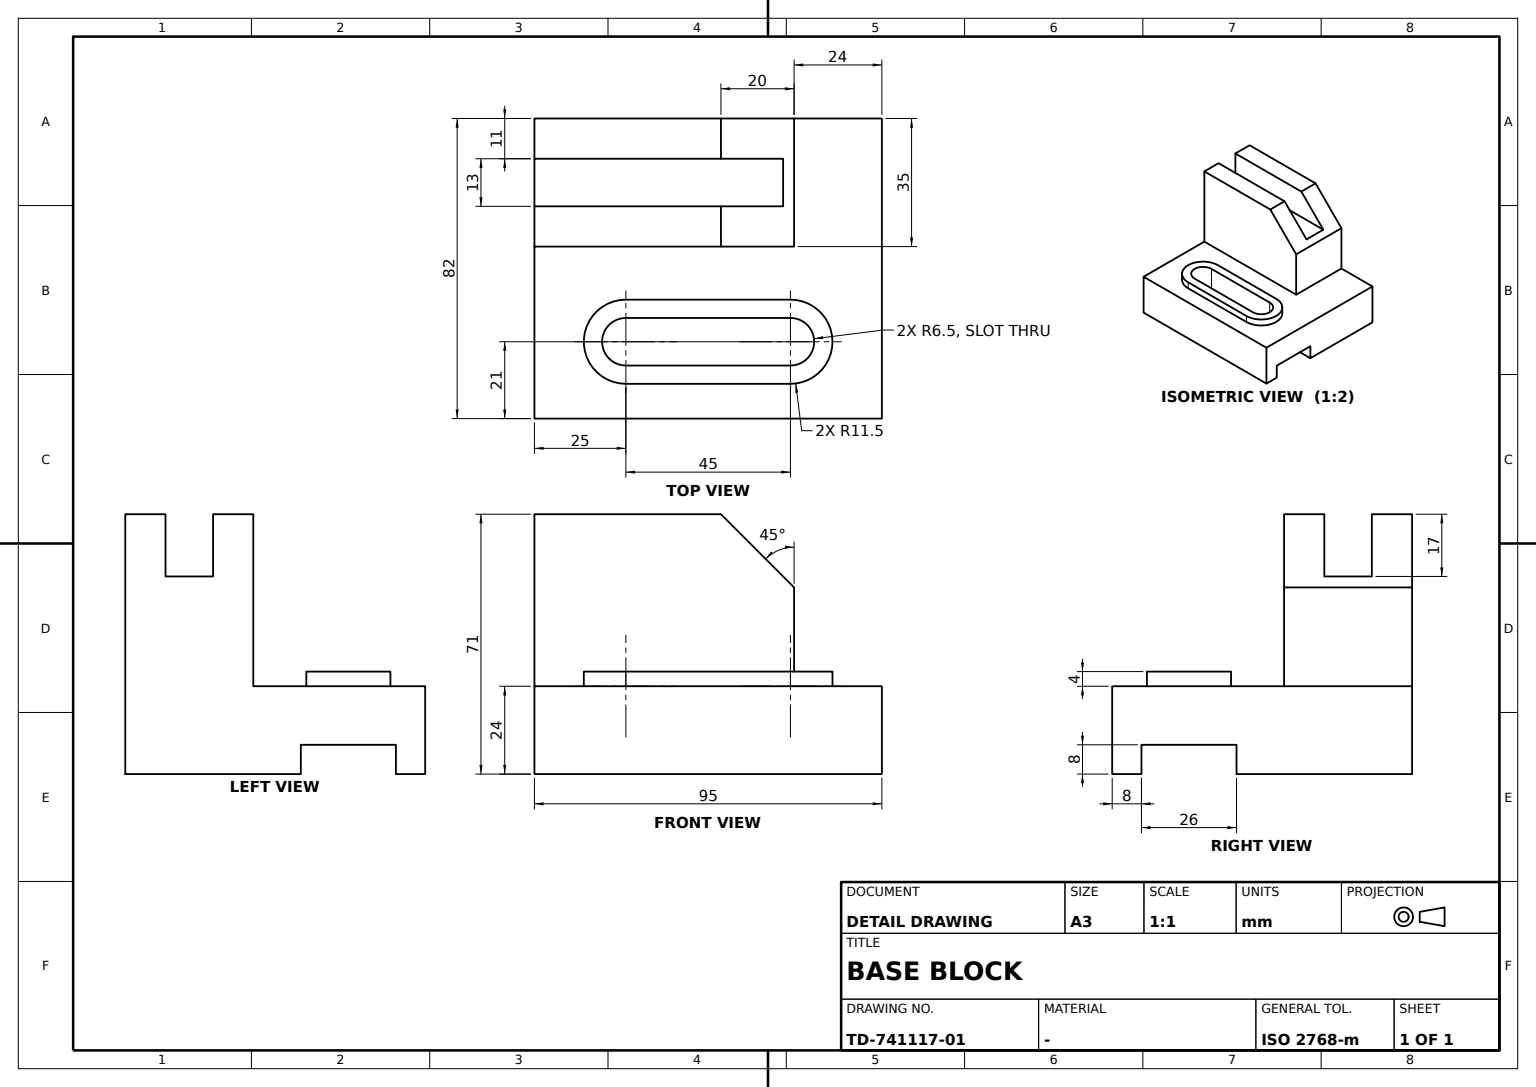
ISO-10303-21;
HEADER;
FILE_DESCRIPTION((''),'2;1');
FILE_NAME('','',(''),(''),'','','');
FILE_SCHEMA(('AUTOMOTIVE_DESIGN'));
ENDSEC;
DATA;
#1=APPLICATION_CONTEXT('');
#2=PRODUCT_CONTEXT('',#1,'mechanical');
#3=PRODUCT('','','',(#2));
#4=PRODUCT_DEFINITION_FORMATION('','',#3);
#5=PRODUCT_DEFINITION_CONTEXT('',#1,'design');
#6=PRODUCT_DEFINITION('','',#4,#5);
#7=PRODUCT_DEFINITION_SHAPE('','',#6);
#8=(LENGTH_UNIT()NAMED_UNIT(*)SI_UNIT(.MILLI.,.METRE.));
#9=(NAMED_UNIT(*)PLANE_ANGLE_UNIT()SI_UNIT($,.RADIAN.));
#10=(NAMED_UNIT(*)SI_UNIT($,.STERADIAN.)SOLID_ANGLE_UNIT());
#11=UNCERTAINTY_MEASURE_WITH_UNIT(LENGTH_MEASURE(0.005),#8,'distance_accuracy_value','');
#12=(GEOMETRIC_REPRESENTATION_CONTEXT(3)GLOBAL_UNCERTAINTY_ASSIGNED_CONTEXT((#11))GLOBAL_UNIT_ASSIGNED_CONTEXT((#8,#9,#10))REPRESENTATION_CONTEXT('',''));
#13=CARTESIAN_POINT('',(95.,34.,8.));
#14=VERTEX_POINT('',#13);
#15=CARTESIAN_POINT('',(0.,34.,8.));
#16=VERTEX_POINT('',#15);
#17=DIRECTION('',(-1.,0.,0.));
#18=VECTOR('',#17,1000.);
#19=LINE('',#15,#18);
#20=EDGE_CURVE('',#14,#16,#19,.T.);
#21=ORIENTED_EDGE('',*,*,#20,.T.);
#22=CARTESIAN_POINT('',(0.,34.,0.));
#23=VERTEX_POINT('',#22);
#24=DIRECTION('',(0.,0.,1.));
#25=VECTOR('',#24,1000.);
#26=LINE('',#22,#25);
#27=EDGE_CURVE('',#23,#16,#26,.T.);
#28=ORIENTED_EDGE('',*,*,#27,.F.);
#29=CARTESIAN_POINT('',(95.,34.,0.));
#30=VERTEX_POINT('',#29);
#31=DIRECTION('',(1.,0.,0.));
#32=VECTOR('',#31,1000.);
#33=LINE('',#22,#32);
#34=EDGE_CURVE('',#23,#30,#33,.T.);
#35=ORIENTED_EDGE('',*,*,#34,.T.);
#36=LINE('',#29,#25);
#37=EDGE_CURVE('',#30,#14,#36,.T.);
#38=ORIENTED_EDGE('',*,*,#37,.T.);
#39=EDGE_LOOP('',(#21,#28,#35,#38));
#40=FACE_BOUND('',#39,.T.);
#41=DIRECTION('',(0.,1.,0.));
#42=AXIS2_PLACEMENT_3D('',#22,#41,#24);
#43=PLANE('',#42);
#44=ADVANCED_FACE('',(#40),#43,.F.);
#45=CARTESIAN_POINT('',(70.,32.5,28.));
#46=VERTEX_POINT('',#45);
#47=CARTESIAN_POINT('',(25.,32.5,28.));
#48=VERTEX_POINT('',#47);
#49=LINE('',#45,#18);
#50=EDGE_CURVE('',#46,#48,#49,.T.);
#51=ORIENTED_EDGE('',*,*,#50,.F.);
#52=CARTESIAN_POINT('',(70.,32.5,24.));
#53=VERTEX_POINT('',#52);
#54=LINE('',#52,#25);
#55=EDGE_CURVE('',#53,#46,#54,.T.);
#56=ORIENTED_EDGE('',*,*,#55,.F.);
#57=CARTESIAN_POINT('',(25.,32.5,24.));
#58=VERTEX_POINT('',#57);
#59=LINE('',#52,#18);
#60=EDGE_CURVE('',#53,#58,#59,.T.);
#61=ORIENTED_EDGE('',*,*,#60,.T.);
#62=LINE('',#57,#25);
#63=EDGE_CURVE('',#58,#48,#62,.T.);
#64=ORIENTED_EDGE('',*,*,#63,.T.);
#65=EDGE_LOOP('',(#51,#56,#61,#64));
#66=FACE_BOUND('',#65,.T.);
#67=AXIS2_PLACEMENT_3D('',#52,#41,#17);
#68=PLANE('',#67);
#69=ADVANCED_FACE('',(#66),#68,.T.);
#70=CARTESIAN_POINT('',(71.,82.,51.));
#71=VERTEX_POINT('',#70);
#72=CARTESIAN_POINT('',(71.,47.,51.));
#73=VERTEX_POINT('',#72);
#74=DIRECTION('',(0.,-1.,0.));
#75=VECTOR('',#74,1000.);
#76=LINE('',#72,#75);
#77=EDGE_CURVE('',#71,#73,#76,.T.);
#78=ORIENTED_EDGE('',*,*,#77,.T.);
#79=CARTESIAN_POINT('',(71.,47.,24.));
#80=VERTEX_POINT('',#79);
#81=LINE('',#79,#25);
#82=EDGE_CURVE('',#80,#73,#81,.T.);
#83=ORIENTED_EDGE('',*,*,#82,.F.);
#84=CARTESIAN_POINT('',(71.,82.,24.));
#85=VERTEX_POINT('',#84);
#86=VECTOR('',#41,1000.);
#87=LINE('',#79,#86);
#88=EDGE_CURVE('',#80,#85,#87,.T.);
#89=ORIENTED_EDGE('',*,*,#88,.T.);
#90=LINE('',#84,#25);
#91=EDGE_CURVE('',#85,#71,#90,.T.);
#92=ORIENTED_EDGE('',*,*,#91,.T.);
#93=EDGE_LOOP('',(#78,#83,#89,#92));
#94=FACE_BOUND('',#93,.T.);
#95=DIRECTION('',(0.,0.,-1.));
#96=AXIS2_PLACEMENT_3D('',#79,#31,#95);
#97=PLANE('',#96);
#98=ADVANCED_FACE('',(#94),#97,.T.);
#99=CARTESIAN_POINT('',(25.,27.5,8.));
#100=VERTEX_POINT('',#99);
#101=CARTESIAN_POINT('',(25.,27.5,28.));
#102=VERTEX_POINT('',#101);
#103=CARTESIAN_POINT('',(25.,27.5,24.));
#104=LINE('',#103,#25);
#105=EDGE_CURVE('',#100,#102,#104,.T.);
#106=ORIENTED_EDGE('',*,*,#105,.T.);
#107=CARTESIAN_POINT('',(25.,14.5,28.));
#108=VERTEX_POINT('',#107);
#109=CARTESIAN_POINT('',(25.,21.,28.));
#110=AXIS2_PLACEMENT_3D('',#109,#95,#41);
#111=CIRCLE('',#110,6.5);
#112=EDGE_CURVE('',#108,#102,#111,.T.);
#113=ORIENTED_EDGE('',*,*,#112,.F.);
#114=CARTESIAN_POINT('',(25.,14.5,8.));
#115=VERTEX_POINT('',#114);
#116=CARTESIAN_POINT('',(25.,14.5,24.));
#117=LINE('',#116,#25);
#118=EDGE_CURVE('',#115,#108,#117,.T.);
#119=ORIENTED_EDGE('',*,*,#118,.F.);
#120=CARTESIAN_POINT('',(25.,21.,8.));
#121=AXIS2_PLACEMENT_3D('',#120,#24,#31);
#122=CIRCLE('',#121,6.5);
#123=EDGE_CURVE('',#100,#115,#122,.T.);
#124=ORIENTED_EDGE('',*,*,#123,.F.);
#125=EDGE_LOOP('',(#106,#113,#119,#124));
#126=FACE_BOUND('',#125,.T.);
#127=CARTESIAN_POINT('',(25.,21.,24.));
#128=AXIS2_PLACEMENT_3D('',#127,#24,#31);
#129=CYLINDRICAL_SURFACE('',#128,6.5);
#130=ADVANCED_FACE('',(#126),#129,.F.);
#131=CARTESIAN_POINT('',(70.,27.5,8.));
#132=VERTEX_POINT('',#131);
#133=CARTESIAN_POINT('',(70.,27.5,28.));
#134=VERTEX_POINT('',#133);
#135=CARTESIAN_POINT('',(70.,27.5,24.));
#136=LINE('',#135,#25);
#137=EDGE_CURVE('',#132,#134,#136,.T.);
#138=ORIENTED_EDGE('',*,*,#137,.F.);
#139=CARTESIAN_POINT('',(76.5,21.,8.));
#140=VERTEX_POINT('',#139);
#141=CARTESIAN_POINT('',(70.,21.,8.));
#142=AXIS2_PLACEMENT_3D('',#141,#24,#31);
#143=CIRCLE('',#142,6.5);
#144=EDGE_CURVE('',#140,#132,#143,.T.);
#145=ORIENTED_EDGE('',*,*,#144,.F.);
#146=CARTESIAN_POINT('',(76.5,21.,28.));
#147=VERTEX_POINT('',#146);
#148=CARTESIAN_POINT('',(76.5,21.,24.));
#149=LINE('',#148,#25);
#150=EDGE_CURVE('',#140,#147,#149,.T.);
#151=ORIENTED_EDGE('',*,*,#150,.T.);
#152=CARTESIAN_POINT('',(70.,21.,28.));
#153=AXIS2_PLACEMENT_3D('',#152,#95,#41);
#154=CIRCLE('',#153,6.5);
#155=EDGE_CURVE('',#134,#147,#154,.T.);
#156=ORIENTED_EDGE('',*,*,#155,.F.);
#157=EDGE_LOOP('',(#138,#145,#151,#156));
#158=FACE_BOUND('',#157,.T.);
#159=CARTESIAN_POINT('',(70.,21.,24.));
#160=AXIS2_PLACEMENT_3D('',#159,#24,#31);
#161=CYLINDRICAL_SURFACE('',#160,6.5);
#162=ADVANCED_FACE('',(#158),#161,.F.);
#163=CARTESIAN_POINT('',(0.,0.,0.));
#164=VERTEX_POINT('',#163);
#165=CARTESIAN_POINT('',(95.,0.,0.));
#166=VERTEX_POINT('',#165);
#167=LINE('',#163,#32);
#168=EDGE_CURVE('',#164,#166,#167,.T.);
#169=ORIENTED_EDGE('',*,*,#168,.T.);
#170=CARTESIAN_POINT('',(95.,0.,24.));
#171=VERTEX_POINT('',#170);
#172=LINE('',#165,#25);
#173=EDGE_CURVE('',#166,#171,#172,.T.);
#174=ORIENTED_EDGE('',*,*,#173,.T.);
#175=CARTESIAN_POINT('',(0.,0.,24.));
#176=VERTEX_POINT('',#175);
#177=LINE('',#175,#32);
#178=EDGE_CURVE('',#176,#171,#177,.T.);
#179=ORIENTED_EDGE('',*,*,#178,.F.);
#180=LINE('',#163,#25);
#181=EDGE_CURVE('',#164,#176,#180,.T.);
#182=ORIENTED_EDGE('',*,*,#181,.F.);
#183=EDGE_LOOP('',(#169,#174,#179,#182));
#184=FACE_BOUND('',#183,.T.);
#185=AXIS2_PLACEMENT_3D('',#163,#74,#95);
#186=PLANE('',#185);
#187=ADVANCED_FACE('',(#184),#186,.T.);
#188=CARTESIAN_POINT('',(51.,47.,71.));
#189=VERTEX_POINT('',#188);
#190=CARTESIAN_POINT('',(49.,47.,73.));
#191=DIRECTION('',(-0.707106781,0.,0.707106781));
#192=VECTOR('',#191,1000.);
#193=LINE('',#190,#192);
#194=EDGE_CURVE('',#73,#189,#193,.T.);
#195=ORIENTED_EDGE('',*,*,#194,.T.);
#196=CARTESIAN_POINT('',(0.,47.,71.));
#197=VERTEX_POINT('',#196);
#198=LINE('',#196,#32);
#199=EDGE_CURVE('',#197,#189,#198,.T.);
#200=ORIENTED_EDGE('',*,*,#199,.F.);
#201=CARTESIAN_POINT('',(0.,47.,24.));
#202=VERTEX_POINT('',#201);
#203=LINE('',#201,#25);
#204=EDGE_CURVE('',#202,#197,#203,.T.);
#205=ORIENTED_EDGE('',*,*,#204,.F.);
#206=LINE('',#201,#32);
#207=EDGE_CURVE('',#202,#80,#206,.T.);
#208=ORIENTED_EDGE('',*,*,#207,.T.);
#209=ORIENTED_EDGE('',*,*,#82,.T.);
#210=EDGE_LOOP('',(#195,#200,#205,#208,#209));
#211=FACE_BOUND('',#210,.T.);
#212=AXIS2_PLACEMENT_3D('',#201,#74,#95);
#213=PLANE('',#212);
#214=ADVANCED_FACE('',(#211),#213,.T.);
#215=CARTESIAN_POINT('',(70.,14.5,28.));
#216=VERTEX_POINT('',#215);
#217=EDGE_CURVE('',#147,#216,#154,.T.);
#218=ORIENTED_EDGE('',*,*,#217,.F.);
#219=ORIENTED_EDGE('',*,*,#150,.F.);
#220=CARTESIAN_POINT('',(70.,14.5,8.));
#221=VERTEX_POINT('',#220);
#222=EDGE_CURVE('',#221,#140,#143,.T.);
#223=ORIENTED_EDGE('',*,*,#222,.F.);
#224=CARTESIAN_POINT('',(70.,14.5,24.));
#225=LINE('',#224,#25);
#226=EDGE_CURVE('',#221,#216,#225,.T.);
#227=ORIENTED_EDGE('',*,*,#226,.T.);
#228=EDGE_LOOP('',(#218,#219,#223,#227));
#229=FACE_BOUND('',#228,.T.);
#230=ADVANCED_FACE('',(#229),#161,.F.);
#231=ORIENTED_EDGE('',*,*,#91,.F.);
#232=CARTESIAN_POINT('',(95.,82.,24.));
#233=VERTEX_POINT('',#232);
#234=LINE('',#232,#18);
#235=EDGE_CURVE('',#233,#85,#234,.T.);
#236=ORIENTED_EDGE('',*,*,#235,.F.);
#237=CARTESIAN_POINT('',(95.,82.,0.));
#238=VERTEX_POINT('',#237);
#239=LINE('',#237,#25);
#240=EDGE_CURVE('',#238,#233,#239,.T.);
#241=ORIENTED_EDGE('',*,*,#240,.F.);
#242=CARTESIAN_POINT('',(0.,82.,0.));
#243=VERTEX_POINT('',#242);
#244=LINE('',#237,#18);
#245=EDGE_CURVE('',#238,#243,#244,.T.);
#246=ORIENTED_EDGE('',*,*,#245,.T.);
#247=CARTESIAN_POINT('',(0.,82.,71.));
#248=VERTEX_POINT('',#247);
#249=LINE('',#242,#25);
#250=EDGE_CURVE('',#243,#248,#249,.T.);
#251=ORIENTED_EDGE('',*,*,#250,.T.);
#252=CARTESIAN_POINT('',(51.,82.,71.));
#253=VERTEX_POINT('',#252);
#254=CARTESIAN_POINT('',(71.,82.,71.));
#255=LINE('',#254,#18);
#256=EDGE_CURVE('',#253,#248,#255,.T.);
#257=ORIENTED_EDGE('',*,*,#256,.F.);
#258=CARTESIAN_POINT('',(108.5,82.,13.5));
#259=DIRECTION('',(0.707106781,0.,-0.707106781));
#260=VECTOR('',#259,1000.);
#261=LINE('',#258,#260);
#262=EDGE_CURVE('',#253,#71,#261,.T.);
#263=ORIENTED_EDGE('',*,*,#262,.T.);
#264=EDGE_LOOP('',(#231,#236,#241,#246,#251,#257,#263));
#265=FACE_BOUND('',#264,.T.);
#266=AXIS2_PLACEMENT_3D('',#237,#41,#24);
#267=PLANE('',#266);
#268=ADVANCED_FACE('',(#265),#267,.T.);
#269=LINE('',#220,#32);
#270=EDGE_CURVE('',#115,#221,#269,.T.);
#271=ORIENTED_EDGE('',*,*,#270,.F.);
#272=ORIENTED_EDGE('',*,*,#118,.T.);
#273=LINE('',#215,#18);
#274=EDGE_CURVE('',#216,#108,#273,.T.);
#275=ORIENTED_EDGE('',*,*,#274,.F.);
#276=ORIENTED_EDGE('',*,*,#226,.F.);
#277=EDGE_LOOP('',(#271,#272,#275,#276));
#278=FACE_BOUND('',#277,.T.);
#279=AXIS2_PLACEMENT_3D('',#224,#41,#17);
#280=PLANE('',#279);
#281=ADVANCED_FACE('',(#278),#280,.T.);
#282=CARTESIAN_POINT('',(0.,8.,0.));
#283=VERTEX_POINT('',#282);
#284=CARTESIAN_POINT('',(95.,8.,0.));
#285=VERTEX_POINT('',#284);
#286=LINE('',#282,#32);
#287=EDGE_CURVE('',#283,#285,#286,.T.);
#288=ORIENTED_EDGE('',*,*,#287,.F.);
#289=CARTESIAN_POINT('',(0.,8.,8.));
#290=VERTEX_POINT('',#289);
#291=VECTOR('',#95,1000.);
#292=LINE('',#289,#291);
#293=EDGE_CURVE('',#290,#283,#292,.T.);
#294=ORIENTED_EDGE('',*,*,#293,.F.);
#295=CARTESIAN_POINT('',(95.,8.,8.));
#296=VERTEX_POINT('',#295);
#297=LINE('',#289,#18);
#298=EDGE_CURVE('',#296,#290,#297,.T.);
#299=ORIENTED_EDGE('',*,*,#298,.F.);
#300=LINE('',#284,#291);
#301=EDGE_CURVE('',#296,#285,#300,.T.);
#302=ORIENTED_EDGE('',*,*,#301,.T.);
#303=EDGE_LOOP('',(#288,#294,#299,#302));
#304=FACE_BOUND('',#303,.T.);
#305=AXIS2_PLACEMENT_3D('',#289,#74,#95);
#306=PLANE('',#305);
#307=ADVANCED_FACE('',(#304),#306,.F.);
#308=CARTESIAN_POINT('',(81.5,21.,28.));
#309=VERTEX_POINT('',#308);
#310=AXIS2_PLACEMENT_3D('',#152,#24,#41);
#311=CIRCLE('',#310,11.5);
#312=EDGE_CURVE('',#309,#46,#311,.T.);
#313=ORIENTED_EDGE('',*,*,#312,.T.);
#314=ORIENTED_EDGE('',*,*,#50,.T.);
#315=CARTESIAN_POINT('',(25.,9.5,28.));
#316=VERTEX_POINT('',#315);
#317=AXIS2_PLACEMENT_3D('',#109,#24,#41);
#318=CIRCLE('',#317,11.5);
#319=EDGE_CURVE('',#48,#316,#318,.T.);
#320=ORIENTED_EDGE('',*,*,#319,.T.);
#321=CARTESIAN_POINT('',(70.,9.5,28.));
#322=VERTEX_POINT('',#321);
#323=LINE('',#315,#32);
#324=EDGE_CURVE('',#316,#322,#323,.T.);
#325=ORIENTED_EDGE('',*,*,#324,.T.);
#326=EDGE_CURVE('',#322,#309,#311,.T.);
#327=ORIENTED_EDGE('',*,*,#326,.T.);
#328=EDGE_LOOP('',(#313,#314,#320,#325,#327));
#329=FACE_BOUND('',#328,.T.);
#330=ORIENTED_EDGE('',*,*,#112,.T.);
#331=LINE('',#101,#32);
#332=EDGE_CURVE('',#102,#134,#331,.T.);
#333=ORIENTED_EDGE('',*,*,#332,.T.);
#334=ORIENTED_EDGE('',*,*,#155,.T.);
#335=ORIENTED_EDGE('',*,*,#217,.T.);
#336=ORIENTED_EDGE('',*,*,#274,.T.);
#337=EDGE_LOOP('',(#330,#333,#334,#335,#336));
#338=FACE_BOUND('',#337,.T.);
#339=AXIS2_PLACEMENT_3D('',#109,#24,#31);
#340=PLANE('',#339);
#341=ADVANCED_FACE('',(#329,#338),#340,.T.);
#342=LINE('',#242,#75);
#343=EDGE_CURVE('',#283,#164,#342,.T.);
#344=ORIENTED_EDGE('',*,*,#343,.T.);
#345=ORIENTED_EDGE('',*,*,#181,.T.);
#346=CARTESIAN_POINT('',(0.,82.,24.));
#347=LINE('',#346,#75);
#348=EDGE_CURVE('',#202,#176,#347,.T.);
#349=ORIENTED_EDGE('',*,*,#348,.F.);
#350=ORIENTED_EDGE('',*,*,#204,.T.);
#351=CARTESIAN_POINT('',(0.,58.,71.));
#352=VERTEX_POINT('',#351);
#353=LINE('',#247,#75);
#354=EDGE_CURVE('',#352,#197,#353,.T.);
#355=ORIENTED_EDGE('',*,*,#354,.F.);
#356=CARTESIAN_POINT('',(0.,58.,54.));
#357=VERTEX_POINT('',#356);
#358=LINE('',#351,#291);
#359=EDGE_CURVE('',#352,#357,#358,.T.);
#360=ORIENTED_EDGE('',*,*,#359,.T.);
#361=CARTESIAN_POINT('',(0.,71.,54.));
#362=VERTEX_POINT('',#361);
#363=LINE('',#356,#86);
#364=EDGE_CURVE('',#357,#362,#363,.T.);
#365=ORIENTED_EDGE('',*,*,#364,.T.);
#366=CARTESIAN_POINT('',(0.,71.,71.));
#367=VERTEX_POINT('',#366);
#368=LINE('',#361,#25);
#369=EDGE_CURVE('',#362,#367,#368,.T.);
#370=ORIENTED_EDGE('',*,*,#369,.T.);
#371=EDGE_CURVE('',#248,#367,#353,.T.);
#372=ORIENTED_EDGE('',*,*,#371,.F.);
#373=ORIENTED_EDGE('',*,*,#250,.F.);
#374=EDGE_CURVE('',#243,#23,#342,.T.);
#375=ORIENTED_EDGE('',*,*,#374,.T.);
#376=ORIENTED_EDGE('',*,*,#27,.T.);
#377=LINE('',#15,#75);
#378=EDGE_CURVE('',#16,#290,#377,.T.);
#379=ORIENTED_EDGE('',*,*,#378,.T.);
#380=ORIENTED_EDGE('',*,*,#293,.T.);
#381=EDGE_LOOP('',(#344,#345,#349,#350,#355,#360,#365,#370,#372,#373,#375,#376,#379,#380));
#382=FACE_BOUND('',#381,.T.);
#383=AXIS2_PLACEMENT_3D('',#242,#17,#24);
#384=PLANE('',#383);
#385=ADVANCED_FACE('',(#382),#384,.T.);
#386=ORIENTED_EDGE('',*,*,#332,.F.);
#387=ORIENTED_EDGE('',*,*,#105,.F.);
#388=LINE('',#99,#18);
#389=EDGE_CURVE('',#132,#100,#388,.T.);
#390=ORIENTED_EDGE('',*,*,#389,.F.);
#391=ORIENTED_EDGE('',*,*,#137,.T.);
#392=EDGE_LOOP('',(#386,#387,#390,#391));
#393=FACE_BOUND('',#392,.T.);
#394=AXIS2_PLACEMENT_3D('',#103,#74,#95);
#395=PLANE('',#394);
#396=ADVANCED_FACE('',(#393),#395,.T.);
#397=LINE('',#165,#86);
#398=EDGE_CURVE('',#30,#238,#397,.T.);
#399=ORIENTED_EDGE('',*,*,#398,.T.);
#400=ORIENTED_EDGE('',*,*,#240,.T.);
#401=LINE('',#170,#86);
#402=EDGE_CURVE('',#171,#233,#401,.T.);
#403=ORIENTED_EDGE('',*,*,#402,.F.);
#404=ORIENTED_EDGE('',*,*,#173,.F.);
#405=EDGE_CURVE('',#166,#285,#397,.T.);
#406=ORIENTED_EDGE('',*,*,#405,.T.);
#407=ORIENTED_EDGE('',*,*,#301,.F.);
#408=CARTESIAN_POINT('',(95.,0.,8.));
#409=LINE('',#408,#75);
#410=EDGE_CURVE('',#14,#296,#409,.T.);
#411=ORIENTED_EDGE('',*,*,#410,.F.);
#412=ORIENTED_EDGE('',*,*,#37,.F.);
#413=EDGE_LOOP('',(#399,#400,#403,#404,#406,#407,#411,#412));
#414=FACE_BOUND('',#413,.T.);
#415=AXIS2_PLACEMENT_3D('',#165,#31,#95);
#416=PLANE('',#415);
#417=ADVANCED_FACE('',(#414),#416,.T.);
#418=ORIENTED_EDGE('',*,*,#168,.F.);
#419=ORIENTED_EDGE('',*,*,#343,.F.);
#420=ORIENTED_EDGE('',*,*,#287,.T.);
#421=ORIENTED_EDGE('',*,*,#405,.F.);
#422=EDGE_LOOP('',(#418,#419,#420,#421));
#423=FACE_BOUND('',#422,.T.);
#424=AXIS2_PLACEMENT_3D('',#163,#24,#31);
#425=PLANE('',#424);
#426=ADVANCED_FACE('',(#423),#425,.F.);
#427=CARTESIAN_POINT('',(25.,9.5,24.));
#428=VERTEX_POINT('',#427);
#429=AXIS2_PLACEMENT_3D('',#127,#24,#41);
#430=CIRCLE('',#429,11.5);
#431=EDGE_CURVE('',#58,#428,#430,.T.);
#432=ORIENTED_EDGE('',*,*,#431,.F.);
#433=ORIENTED_EDGE('',*,*,#60,.F.);
#434=CARTESIAN_POINT('',(81.5,21.,24.));
#435=VERTEX_POINT('',#434);
#436=AXIS2_PLACEMENT_3D('',#159,#24,#41);
#437=CIRCLE('',#436,11.5);
#438=EDGE_CURVE('',#435,#53,#437,.T.);
#439=ORIENTED_EDGE('',*,*,#438,.F.);
#440=CARTESIAN_POINT('',(70.,9.5,24.));
#441=VERTEX_POINT('',#440);
#442=EDGE_CURVE('',#441,#435,#437,.T.);
#443=ORIENTED_EDGE('',*,*,#442,.F.);
#444=LINE('',#427,#32);
#445=EDGE_CURVE('',#428,#441,#444,.T.);
#446=ORIENTED_EDGE('',*,*,#445,.F.);
#447=EDGE_LOOP('',(#432,#433,#439,#443,#446));
#448=FACE_BOUND('',#447,.T.);
#449=ORIENTED_EDGE('',*,*,#348,.T.);
#450=ORIENTED_EDGE('',*,*,#178,.T.);
#451=ORIENTED_EDGE('',*,*,#402,.T.);
#452=ORIENTED_EDGE('',*,*,#235,.T.);
#453=ORIENTED_EDGE('',*,*,#88,.F.);
#454=ORIENTED_EDGE('',*,*,#207,.F.);
#455=EDGE_LOOP('',(#449,#450,#451,#452,#453,#454));
#456=FACE_BOUND('',#455,.T.);
#457=AXIS2_PLACEMENT_3D('',#175,#24,#31);
#458=PLANE('',#457);
#459=ADVANCED_FACE('',(#448,#456),#458,.T.);
#460=LINE('',#434,#25);
#461=EDGE_CURVE('',#435,#309,#460,.T.);
#462=ORIENTED_EDGE('',*,*,#461,.F.);
#463=ORIENTED_EDGE('',*,*,#438,.T.);
#464=ORIENTED_EDGE('',*,*,#55,.T.);
#465=ORIENTED_EDGE('',*,*,#312,.F.);
#466=EDGE_LOOP('',(#462,#463,#464,#465));
#467=FACE_BOUND('',#466,.T.);
#468=CYLINDRICAL_SURFACE('',#160,11.5);
#469=ADVANCED_FACE('',(#467),#468,.T.);
#470=ORIENTED_EDGE('',*,*,#319,.F.);
#471=ORIENTED_EDGE('',*,*,#63,.F.);
#472=ORIENTED_EDGE('',*,*,#431,.T.);
#473=LINE('',#427,#25);
#474=EDGE_CURVE('',#428,#316,#473,.T.);
#475=ORIENTED_EDGE('',*,*,#474,.T.);
#476=EDGE_LOOP('',(#470,#471,#472,#475));
#477=FACE_BOUND('',#476,.T.);
#478=CYLINDRICAL_SURFACE('',#128,11.5);
#479=ADVANCED_FACE('',(#477),#478,.T.);
#480=ORIENTED_EDGE('',*,*,#194,.F.);
#481=ORIENTED_EDGE('',*,*,#77,.F.);
#482=ORIENTED_EDGE('',*,*,#262,.F.);
#483=CARTESIAN_POINT('',(51.,71.,71.));
#484=VERTEX_POINT('',#483);
#485=CARTESIAN_POINT('',(51.,0.,71.));
#486=LINE('',#485,#86);
#487=EDGE_CURVE('',#484,#253,#486,.T.);
#488=ORIENTED_EDGE('',*,*,#487,.F.);
#489=CARTESIAN_POINT('',(68.,71.,54.));
#490=VERTEX_POINT('',#489);
#491=LINE('',#483,#192);
#492=EDGE_CURVE('',#490,#484,#491,.T.);
#493=ORIENTED_EDGE('',*,*,#492,.F.);
#494=CARTESIAN_POINT('',(68.,58.,54.));
#495=VERTEX_POINT('',#494);
#496=CARTESIAN_POINT('',(68.,0.,54.));
#497=LINE('',#496,#86);
#498=EDGE_CURVE('',#495,#490,#497,.T.);
#499=ORIENTED_EDGE('',*,*,#498,.F.);
#500=CARTESIAN_POINT('',(51.,58.,71.));
#501=VERTEX_POINT('',#500);
#502=LINE('',#500,#260);
#503=EDGE_CURVE('',#501,#495,#502,.T.);
#504=ORIENTED_EDGE('',*,*,#503,.F.);
#505=EDGE_CURVE('',#189,#501,#486,.T.);
#506=ORIENTED_EDGE('',*,*,#505,.F.);
#507=EDGE_LOOP('',(#480,#481,#482,#488,#493,#499,#504,#506));
#508=FACE_BOUND('',#507,.T.);
#509=DIRECTION('',(-0.707106781,0.,-0.707106781));
#510=AXIS2_PLACEMENT_3D('',#485,#509,#41);
#511=PLANE('',#510);
#512=ADVANCED_FACE('',(#508),#511,.F.);
#513=ORIENTED_EDGE('',*,*,#498,.T.);
#514=LINE('',#361,#18);
#515=EDGE_CURVE('',#490,#362,#514,.T.);
#516=ORIENTED_EDGE('',*,*,#515,.T.);
#517=ORIENTED_EDGE('',*,*,#364,.F.);
#518=LINE('',#356,#18);
#519=EDGE_CURVE('',#495,#357,#518,.T.);
#520=ORIENTED_EDGE('',*,*,#519,.F.);
#521=EDGE_LOOP('',(#513,#516,#517,#520));
#522=FACE_BOUND('',#521,.T.);
#523=AXIS2_PLACEMENT_3D('',#356,#95,#17);
#524=PLANE('',#523);
#525=ADVANCED_FACE('',(#522),#524,.F.);
#526=ORIENTED_EDGE('',*,*,#487,.T.);
#527=ORIENTED_EDGE('',*,*,#256,.T.);
#528=ORIENTED_EDGE('',*,*,#371,.T.);
#529=LINE('',#366,#32);
#530=EDGE_CURVE('',#367,#484,#529,.T.);
#531=ORIENTED_EDGE('',*,*,#530,.T.);
#532=EDGE_LOOP('',(#526,#527,#528,#531));
#533=FACE_BOUND('',#532,.T.);
#534=CARTESIAN_POINT('',(0.,0.,71.));
#535=AXIS2_PLACEMENT_3D('',#534,#24,#31);
#536=PLANE('',#535);
#537=ADVANCED_FACE('',(#533),#536,.T.);
#538=LINE('',#440,#25);
#539=EDGE_CURVE('',#441,#322,#538,.T.);
#540=ORIENTED_EDGE('',*,*,#539,.F.);
#541=ORIENTED_EDGE('',*,*,#442,.T.);
#542=ORIENTED_EDGE('',*,*,#461,.T.);
#543=ORIENTED_EDGE('',*,*,#326,.F.);
#544=EDGE_LOOP('',(#540,#541,#542,#543));
#545=FACE_BOUND('',#544,.T.);
#546=ADVANCED_FACE('',(#545),#468,.T.);
#547=ORIENTED_EDGE('',*,*,#474,.F.);
#548=ORIENTED_EDGE('',*,*,#445,.T.);
#549=ORIENTED_EDGE('',*,*,#539,.T.);
#550=ORIENTED_EDGE('',*,*,#324,.F.);
#551=EDGE_LOOP('',(#547,#548,#549,#550));
#552=FACE_BOUND('',#551,.T.);
#553=AXIS2_PLACEMENT_3D('',#427,#74,#31);
#554=PLANE('',#553);
#555=ADVANCED_FACE('',(#552),#554,.T.);
#556=ORIENTED_EDGE('',*,*,#378,.F.);
#557=ORIENTED_EDGE('',*,*,#20,.F.);
#558=ORIENTED_EDGE('',*,*,#410,.T.);
#559=ORIENTED_EDGE('',*,*,#298,.T.);
#560=EDGE_LOOP('',(#556,#557,#558,#559));
#561=FACE_BOUND('',#560,.T.);
#562=ORIENTED_EDGE('',*,*,#389,.T.);
#563=ORIENTED_EDGE('',*,*,#123,.T.);
#564=ORIENTED_EDGE('',*,*,#270,.T.);
#565=ORIENTED_EDGE('',*,*,#222,.T.);
#566=ORIENTED_EDGE('',*,*,#144,.T.);
#567=EDGE_LOOP('',(#562,#563,#564,#565,#566));
#568=FACE_BOUND('',#567,.T.);
#569=AXIS2_PLACEMENT_3D('',#15,#24,#31);
#570=PLANE('',#569);
#571=ADVANCED_FACE('',(#561,#568),#570,.F.);
#572=ORIENTED_EDGE('',*,*,#515,.F.);
#573=ORIENTED_EDGE('',*,*,#492,.T.);
#574=ORIENTED_EDGE('',*,*,#530,.F.);
#575=ORIENTED_EDGE('',*,*,#369,.F.);
#576=EDGE_LOOP('',(#572,#573,#574,#575));
#577=FACE_BOUND('',#576,.T.);
#578=AXIS2_PLACEMENT_3D('',#361,#41,#24);
#579=PLANE('',#578);
#580=ADVANCED_FACE('',(#577),#579,.F.);
#581=ORIENTED_EDGE('',*,*,#199,.T.);
#582=ORIENTED_EDGE('',*,*,#505,.T.);
#583=LINE('',#351,#32);
#584=EDGE_CURVE('',#352,#501,#583,.T.);
#585=ORIENTED_EDGE('',*,*,#584,.F.);
#586=ORIENTED_EDGE('',*,*,#354,.T.);
#587=EDGE_LOOP('',(#581,#582,#585,#586));
#588=FACE_BOUND('',#587,.T.);
#589=ADVANCED_FACE('',(#588),#536,.T.);
#590=ORIENTED_EDGE('',*,*,#584,.T.);
#591=ORIENTED_EDGE('',*,*,#503,.T.);
#592=ORIENTED_EDGE('',*,*,#519,.T.);
#593=ORIENTED_EDGE('',*,*,#359,.F.);
#594=EDGE_LOOP('',(#590,#591,#592,#593));
#595=FACE_BOUND('',#594,.T.);
#596=AXIS2_PLACEMENT_3D('',#351,#74,#95);
#597=PLANE('',#596);
#598=ADVANCED_FACE('',(#595),#597,.F.);
#599=ORIENTED_EDGE('',*,*,#398,.F.);
#600=ORIENTED_EDGE('',*,*,#34,.F.);
#601=ORIENTED_EDGE('',*,*,#374,.F.);
#602=ORIENTED_EDGE('',*,*,#245,.F.);
#603=EDGE_LOOP('',(#599,#600,#601,#602));
#604=FACE_BOUND('',#603,.T.);
#605=ADVANCED_FACE('',(#604),#425,.F.);
#606=CLOSED_SHELL('',(#44,#69,#98,#130,#162,#187,#214,#230,#268,#281,#307,#341,#385,#396,#417,#426,#459,#469,#479,#512,#525,#537,#546,#555,#571,#580,#589,#598,#605));
#607=MANIFOLD_SOLID_BREP('',#606);
#608=ADVANCED_BREP_SHAPE_REPRESENTATION('',(#607),#12);
#609=SHAPE_DEFINITION_REPRESENTATION(#7,#608);
ENDSEC;
END-ISO-10303-21;
